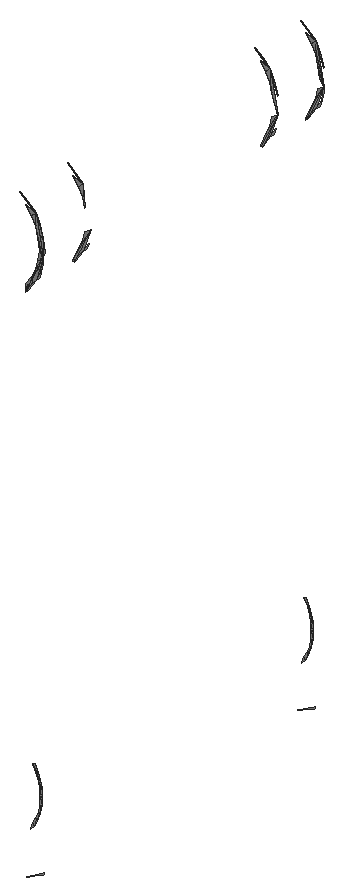
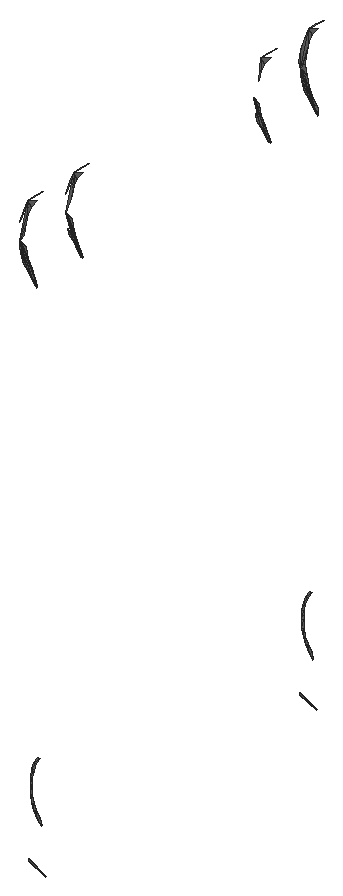
# SketchUp Ruby script. Lengths in inches.
U = 1.inch
M = Sketchup.active_model
def pt(a) = Geom::Point3d.new(a.map { |v| v * U })
def face(e, loops, mat)
  f = e.add_face(loops[0].map { |a| pt(a) })
  loops[1..].each { |l| e.add_face(l.map { |a| pt(a) }).erase! }
  f.material = f.back_material = mat if mat
  f
end
# faces: each face lists its corners as indices into pts; further lists are holes
def faces(e, pts, list, mat = nil) = list.each { |f| face(e, (f[0].is_a?(Array) ? f : [f]).map { |l| l.map { |i| pts[i] } }, mat) }
# xy, xz, yz: faces in a plane at the given z, y or x. An outline is a flat list of corners, or four numbers for a rectangle; further outlines are holes
def ring(l) = l.size == 4 ? [[l[0], l[1]], [l[2], l[1]], [l[2], l[3]], [l[0], l[3]]] : l.each_slice(2).to_a
def flat(e, list, mat, &to3) = list.each { |f| face(e, (f[0].is_a?(Array) ? f : [f]).map { |l| ring(l).map { |u, v| to3.(u, v) } }, mat) }
def xy(e, z, list, mat = nil) = flat(e, list, mat) { |x, y| [x, y, z] }
def xz(e, y, list, mat = nil) = flat(e, list, mat) { |x, z| [x, y, z] }
def yz(e, x, list, mat = nil) = flat(e, list, mat) { |y, z| [x, y, z] }
def lines(e, pts, list) = list.each { |a, b| e.add_line(pt(pts[a]), pt(pts[b])) }
# prism: a flat outline (further loops are holes) pulled along v
def prism(e, loops, v, mat = nil)
  f = face(e, loops, mat); d = Geom::Vector3d.new(v.map { |x| x * U })
  f.pushpull(f.normal.samedirection?(d) ? d.length : -d.length)
end
def box(e, o, s, mat = nil) = prism(e, [[o, [o[0] + s[0], o[1], o[2]], [o[0] + s[0], o[1] + s[1], o[2]], [o[0], o[1] + s[1], o[2]]]], [0, 0, s[2]], mat)
def at(x, y, z, deg = 0) = Geom::Transformation.translation(pt([x, y, z])) * Geom::Transformation.rotation(ORIGIN, Z_AXIS, deg.degrees)
def axes(o, x, y, z) = Geom::Transformation.new([*x, 0, *y, 0, *z, 0, *pt(o).to_a, 1])
def part(name) = M.definitions.add(name)
# library, detail: a bought-in or finely detailed component or shape, given as its bounding box
def library(name, o, s) = part(name).tap { |d| box(d.entities, o, s) }
def detail(e, o, s) = box(e.add_group.entities, o, s)
def put(e, d, t, mat = nil) = e.add_instance(d, t).tap { |i| i.material = mat if mat }
def group(e, t, mat = nil) = e.add_group.tap { |g| g.transformation = t; g.material = mat if mat }.entities
root = M.entities
M.materials.add("Material \#1").color = [140, 140, 140]
xz(root,115.821,[[101.517,193.523,101.516,193.583,101.519,193.535],[101.519,193.535,101.516,193.583,101.546,193.619],[101.519,193.535,101.546,193.619,101.523,193.546],[101.523,193.546,101.546,193.619,101.57,193.662],[101.523,193.546,101.57,193.662,101.614,193.729],
  [101.523,193.546,101.614,193.729,101.525,193.55],[101.525,193.55,101.614,193.729,101.529,193.555],[101.529,193.555,101.571,193.607,101.533,193.559],[101.529,193.555,101.614,193.729,101.571,193.607],[101.533,193.559,101.571,193.607,101.553,193.582],
  [101.571,193.607,101.599,193.665,101.586,193.635],[101.571,193.607,101.614,193.729,101.599,193.665],[101.57,193.662,101.584,193.711,101.614,193.729],[101.599,193.665,101.614,193.729,101.608,193.696],[101.584,193.711,101.59,193.764,101.614,193.729],
  [101.614,193.729,101.567,193.929,101.61,193.824],[101.614,193.729,101.57,193.866,101.567,193.929],[101.614,193.729,101.584,193.817,101.57,193.866],[101.614,193.729,101.59,193.764,101.584,193.817],[101.614,193.729,101.61,193.824,101.616,193.764],
  [101.61,193.824,101.567,193.929,101.593,193.88],[101.57,193.866,101.546,193.909,101.567,193.929],[101.546,193.909,101.516,193.945,101.567,193.929],[101.567,193.929,101.491,194.001,101.532,193.969]],"Material \#1")
xz(root,115.852,[[101.496,190.774,101.589,190.816,101.593,190.805],[101.516,190.997,101.531,191.032,101.539,191.024],[101.539,191.024,101.531,191.032,101.549,191.062],[101.539,191.024,101.549,191.062,101.557,191.056],[101.557,191.056,101.549,191.062,101.562,191.095],
  [101.557,191.056,101.562,191.095,101.571,191.091],[101.571,191.091,101.562,191.095,101.571,191.131],[101.571,191.091,101.571,191.131,101.58,191.129],[101.58,191.129,101.571,191.131,101.574,191.169],[101.58,191.129,101.574,191.169,101.583,191.169],
  [101.574,191.169,101.571,191.207,101.583,191.169],[101.583,191.169,101.571,191.207,101.58,191.21],[101.571,191.207,101.562,191.244,101.58,191.21],[101.58,191.21,101.562,191.244,101.571,191.248],[101.562,191.244,101.549,191.277,101.571,191.248],
  [101.571,191.248,101.549,191.277,101.557,191.283],[101.549,191.277,101.531,191.307,101.557,191.283],[101.557,191.283,101.531,191.307,101.539,191.314]],"Material \#1")
xz(root,116.128,[[101.523,193.546,101.525,193.55,101.614,193.729],[101.523,193.546,101.614,193.729,101.546,193.619],[101.525,193.55,101.529,193.555,101.614,193.729],[101.529,193.555,101.533,193.559,101.571,193.607],[101.529,193.555,101.571,193.607,101.614,193.729],
  [101.533,193.559,101.553,193.582,101.571,193.607],[101.571,193.607,101.586,193.635,101.599,193.665],[101.546,193.619,101.614,193.729,101.57,193.662],[101.57,193.662,101.614,193.729,101.584,193.711],[101.584,193.817,101.567,193.929,101.57,193.866],
  [101.57,193.866,101.567,193.929,101.546,193.909],[101.546,193.909,101.567,193.929,101.516,193.945],[101.567,193.929,101.532,193.969,101.491,194.001]],"Material \#1")
xz(root,117.355,[[101.523,193.546,101.546,193.619,101.614,193.729],[101.523,193.546,101.614,193.729,101.525,193.55],[101.525,193.55,101.614,193.729,101.529,193.555],[101.529,193.555,101.571,193.607,101.533,193.559],[101.529,193.555,101.614,193.729,101.571,193.607],
  [101.533,193.559,101.571,193.607,101.553,193.582],[101.571,193.607,101.599,193.665,101.586,193.635],[101.546,193.619,101.57,193.662,101.614,193.729],[101.57,193.662,101.584,193.711,101.614,193.729],[101.614,193.729,101.584,193.817,101.567,193.929],
  [101.584,193.817,101.57,193.866,101.567,193.929],[101.61,193.824,101.567,193.929,101.593,193.88],[101.57,193.866,101.546,193.909,101.567,193.929],[101.546,193.909,101.516,193.945,101.567,193.929],[101.567,193.929,101.491,194.001,101.532,193.969]],"Material \#1")
xz(root,117.632,[[101.496,190.774,101.593,190.805,101.589,190.816],[101.516,190.997,101.539,191.024,101.531,191.032],[101.539,191.024,101.549,191.062,101.531,191.032],[101.539,191.024,101.557,191.056,101.549,191.062],[101.557,191.056,101.562,191.095,101.549,191.062],
  [101.557,191.056,101.571,191.091,101.562,191.095],[101.571,191.091,101.571,191.131,101.562,191.095],[101.571,191.091,101.58,191.129,101.571,191.131],[101.58,191.129,101.574,191.169,101.571,191.131],[101.58,191.129,101.583,191.169,101.574,191.169],
  [101.574,191.169,101.583,191.169,101.571,191.207],[101.583,191.169,101.58,191.21,101.571,191.207],[101.571,191.207,101.58,191.21,101.562,191.244],[101.58,191.21,101.571,191.248,101.562,191.244],[101.562,191.244,101.571,191.248,101.549,191.277],
  [101.571,191.248,101.557,191.283,101.549,191.277],[101.549,191.277,101.557,191.283,101.531,191.307],[101.557,191.283,101.539,191.314,101.531,191.307]],"Material \#1")
xz(root,117.662,[[101.519,193.535,101.523,193.546,101.546,193.619],[101.523,193.546,101.525,193.55,101.614,193.729],[101.523,193.546,101.57,193.662,101.546,193.619],[101.523,193.546,101.614,193.729,101.57,193.662],[101.525,193.55,101.529,193.555,101.614,193.729],
  [101.529,193.555,101.533,193.559,101.571,193.607],[101.529,193.555,101.571,193.607,101.614,193.729],[101.533,193.559,101.553,193.582,101.571,193.607],[101.571,193.607,101.586,193.635,101.599,193.665],[101.57,193.662,101.614,193.729,101.584,193.711],
  [101.599,193.665,101.608,193.696,101.614,193.729],[101.614,193.729,101.567,193.929,101.57,193.866],[101.614,193.729,101.57,193.866,101.584,193.817],[101.614,193.729,101.584,193.817,101.59,193.764],[101.61,193.824,101.593,193.88,101.567,193.929],
  [101.57,193.866,101.567,193.929,101.546,193.909],[101.546,193.909,101.567,193.929,101.516,193.945],[101.567,193.929,101.532,193.969,101.491,194.001]],"Material \#1")
